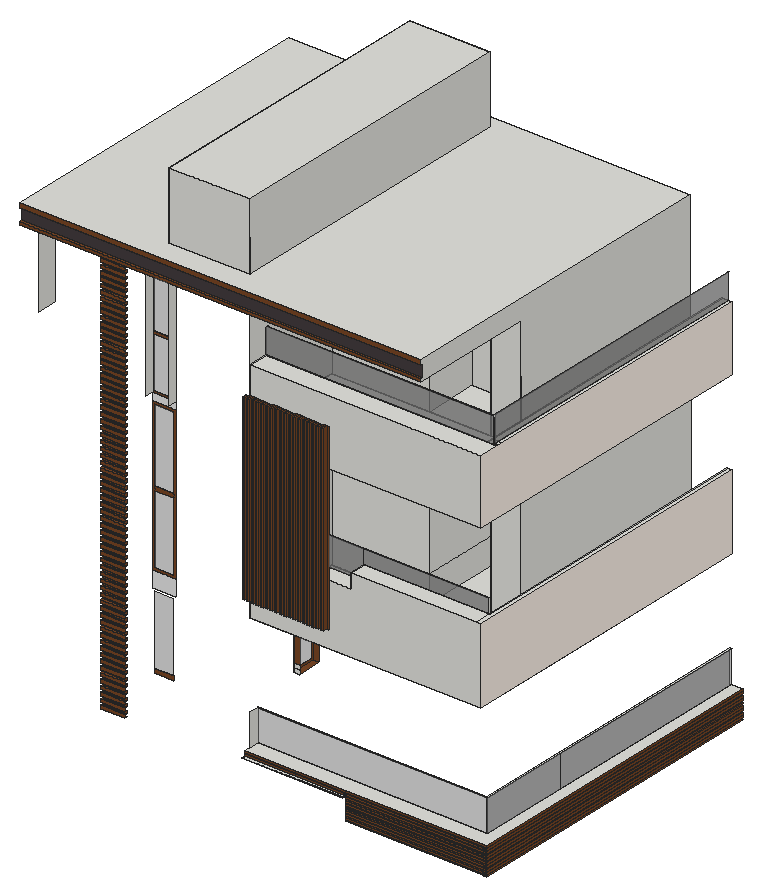
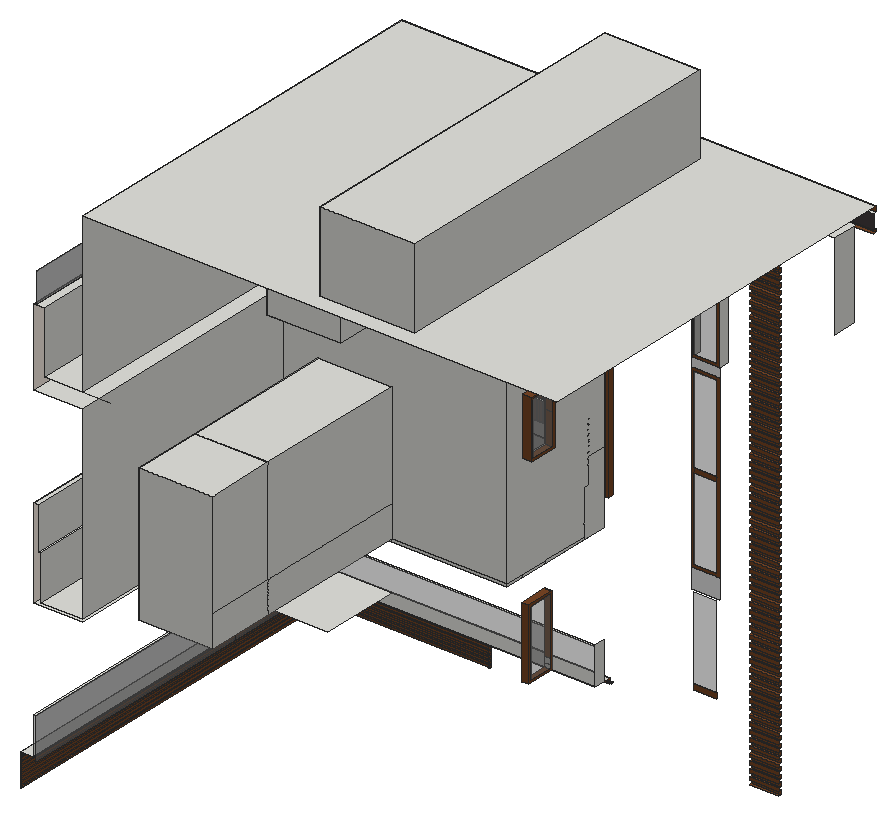
# SketchUp Ruby script. Lengths in inches.
U = 1.inch
M = Sketchup.active_model
def pt(a) = Geom::Point3d.new(a.map { |v| v * U })
def face(e, loops, mat)
  f = e.add_face(loops[0].map { |a| pt(a) })
  loops[1..].each { |l| e.add_face(l.map { |a| pt(a) }).erase! }
  f.material = f.back_material = mat if mat
  f
end
# faces: each face lists its corners as indices into pts; further lists are holes
def faces(e, pts, list, mat = nil) = list.each { |f| face(e, (f[0].is_a?(Array) ? f : [f]).map { |l| l.map { |i| pts[i] } }, mat) }
# xy, xz, yz: faces in a plane at the given z, y or x. An outline is a flat list of corners, or four numbers for a rectangle; further outlines are holes
def ring(l) = l.size == 4 ? [[l[0], l[1]], [l[2], l[1]], [l[2], l[3]], [l[0], l[3]]] : l.each_slice(2).to_a
def flat(e, list, mat, &to3) = list.each { |f| face(e, (f[0].is_a?(Array) ? f : [f]).map { |l| ring(l).map { |u, v| to3.(u, v) } }, mat) }
def xy(e, z, list, mat = nil) = flat(e, list, mat) { |x, y| [x, y, z] }
def xz(e, y, list, mat = nil) = flat(e, list, mat) { |x, z| [x, y, z] }
def yz(e, x, list, mat = nil) = flat(e, list, mat) { |y, z| [x, y, z] }
def lines(e, pts, list) = list.each { |a, b| e.add_line(pt(pts[a]), pt(pts[b])) }
# prism: a flat outline (further loops are holes) pulled along v
def prism(e, loops, v, mat = nil)
  f = face(e, loops, mat); d = Geom::Vector3d.new(v.map { |x| x * U })
  f.pushpull(f.normal.samedirection?(d) ? d.length : -d.length)
end
def box(e, o, s, mat = nil) = prism(e, [[o, [o[0] + s[0], o[1], o[2]], [o[0] + s[0], o[1] + s[1], o[2]], [o[0], o[1] + s[1], o[2]]]], [0, 0, s[2]], mat)
def at(x, y, z, deg = 0) = Geom::Transformation.translation(pt([x, y, z])) * Geom::Transformation.rotation(ORIGIN, Z_AXIS, deg.degrees)
def axes(o, x, y, z) = Geom::Transformation.new([*x, 0, *y, 0, *z, 0, *pt(o).to_a, 1])
def part(name) = M.definitions.add(name)
# library, detail: a bought-in or finely detailed component or shape, given as its bounding box
def library(name, o, s) = part(name).tap { |d| box(d.entities, o, s) }
def detail(e, o, s) = box(e.add_group.entities, o, s)
def put(e, d, t, mat = nil) = e.add_instance(d, t).tap { |i| i.material = mat if mat }
def group(e, t, mat = nil) = e.add_group.tap { |g| g.transformation = t; g.material = mat if mat }.entities
root = M.entities
M.materials.add("[0009_Linen]").color = [250, 240, 230]
M.materials.add("[Asphalt New]").color = [67, 60, 62]
M.materials.add("[Polished Concrete Old]").color = [229, 229, 229]
M.materials.add("[Translucent Glass Gray]").color = [128, 128, 128]
M.materials["[Translucent Glass Gray]"].alpha = 0.5
M.materials.add("[Wood Veneer 01]").color = [120, 70, 37]
xy(root,339.5,[[701.8,342.29,960.69,342.73],[960.69,342.73,962.51,934.03]],"[Wood Veneer 01]")
xy(root,342.02,[[701.8,342.29,960.69,342.73],[960.69,342.73,962.51,934.03]],"[Wood Veneer 01]")
xy(root,343.69,[[224.18,374.04,268.36,378.04]],"[Wood Veneer 01]")
xy(root,345.19,[[701.8,342.29,960.69,342.73],[960.69,342.73,962.51,934.03]],"[Wood Veneer 01]")
xy(root,347.71,[[701.8,342.29,960.69,342.73],[960.69,342.73,962.51,934.03]],"[Wood Veneer 01]")
xy(root,349.71,[[224.18,374.04,268.36,378.04]],"[Wood Veneer 01]")
xy(root,350.88,[[701.8,342.29,960.69,342.73],[960.69,342.73,962.51,934.03]],"[Wood Veneer 01]")
xy(root,353.39,[[701.8,342.29,960.69,342.73],[960.69,342.73,962.51,934.03]],"[Wood Veneer 01]")
xy(root,354.57,[[224.18,374.04,268.36,378.04]],"[Wood Veneer 01]")
xy(root,356.57,[[701.8,342.29,960.69,342.73],[960.69,342.73,962.51,934.03]],"[Wood Veneer 01]")
xy(root,359.08,[[701.8,342.29,960.69,342.73],[960.69,342.73,962.51,934.03]],"[Wood Veneer 01]")
xy(root,360.59,[[224.18,374.04,268.36,378.04]],"[Wood Veneer 01]")
xy(root,362.25,[[701.8,342.29,960.69,342.73],[960.69,342.73,962.51,934.03]],"[Wood Veneer 01]")
xy(root,364.77,[[701.8,342.29,960.69,342.73],[960.69,342.73,962.51,934.03]],"[Wood Veneer 01]")
xy(root,365.44,[[224.18,374.04,268.36,378.04]],"[Wood Veneer 01]")
xy(root,367.94,[[701.8,342.29,960.69,342.73],[960.69,342.73,962.51,934.03]],"[Wood Veneer 01]")
xy(root,370.46,[[701.8,342.29,960.69,342.73],[960.69,342.73,962.51,934.03]],"[Wood Veneer 01]")
xy(root,371.46,[[224.18,374.04,268.36,378.04]],"[Wood Veneer 01]")
xy(root,373.63,[[701.8,342.29,960.69,342.73],[960.69,342.73,962.51,934.03]],"[Wood Veneer 01]")
xy(root,376.14,[[701.8,342.29,960.69,342.73],[960.69,342.73,962.51,934.03]],"[Wood Veneer 01]")
xy(root,376.32,[[224.18,374.04,268.36,378.04]],"[Wood Veneer 01]")
xy(root,379.32,[[701.8,342.29,960.69,342.73],[960.69,342.73,962.51,934.03]],"[Wood Veneer 01]")
xy(root,380.42,[[515.24,336.73,701.8,339.61]])
xy(root,381.83,[[515.24,336.73,701.8,342.29]])
xy(root,381.83,[[701.8,342.29,960.69,342.73],[960.69,342.73,962.51,934.03]],"[Wood Veneer 01]")
xy(root,382.34,[[224.18,374.04,268.36,378.04]],"[Wood Veneer 01]")
xy(root,385,[[515.24,342.29,701.8,342.73],[701.8,342.29,960.69,342.73],[960.69,342.73,962.51,934.03]],"[Wood Veneer 01]")
xy(root,386.71,[[515.24,342.29,701.8,342.73],[701.8,342.29,962.51,342.73],[960.69,342.73,962.51,934.03]],"[Wood Veneer 01]")
xy(root,387.19,[[224.18,374.04,268.36,378.04]],"[Wood Veneer 01]")
xy(root,390.25,[[515.24,342.29,962.51,342.29,962.51,934.03,941.71,934.03,941.71,371.82,515.24,371.82]])
xy(root,393.21,[[224.18,374.04,268.36,378.04]],"[Wood Veneer 01]")
xy(root,398.07,[[224.18,374.04,268.36,378.04]],"[Wood Veneer 01]")
xy(root,404.09,[[224.18,374.04,268.36,378.04]],"[Wood Veneer 01]")
xy(root,408.94,[[224.18,374.04,268.36,378.04]],"[Wood Veneer 01]")
xy(root,414.96,[[224.18,374.04,268.36,378.04]],"[Wood Veneer 01]")
xy(root,419.82,[[224.18,374.04,268.36,378.04]],"[Wood Veneer 01]")
xy(root,425.84,[[224.18,374.04,268.36,378.04]],"[Wood Veneer 01]")
xy(root,430.69,[[224.18,374.04,268.36,378.04]],"[Wood Veneer 01]")
xy(root,436.71,[[224.18,374.04,268.36,378.04]],"[Wood Veneer 01]")
xy(root,441.57,[[224.18,374.04,268.36,378.04]],"[Wood Veneer 01]")
xy(root,447.59,[[224.18,374.04,268.36,378.04]],"[Wood Veneer 01]")
xy(root,449.0625,[[515.24,371.82,941.71,371.82,941.71,934.03,937.99,934.03,937.99,373.53,515.24,373.53]])
xy(root,452.44,[[224.18,374.04,268.36,378.04]],"[Wood Veneer 01]")
xy(root,458.46,[[224.18,374.04,268.36,378.04]],"[Wood Veneer 01]")
xy(root,461.11,[[504.05,469.55,515.24,514.92]],"[Wood Veneer 01]")
xy(root,463.32,[[224.18,374.04,268.36,378.04]],"[Wood Veneer 01]")
xy(root,469.34,[[224.18,374.04,268.36,378.04]],"[Wood Veneer 01]")
xy(root,474.19,[[224.18,374.04,268.36,378.04]],"[Wood Veneer 01]")
xy(root,480.21,[[224.18,374.04,268.36,378.04]],"[Wood Veneer 01]")
xy(root,485.07,[[224.18,374.04,268.36,378.04]],"[Wood Veneer 01]")
xy(root,491.09,[[224.18,374.04,268.36,378.04]],"[Wood Veneer 01]")
xy(root,495.94,[[224.18,374.04,268.36,378.04]],"[Wood Veneer 01]")
xy(root,501.96,[[224.18,374.04,268.36,378.04]],"[Wood Veneer 01]")
xy(root,507.44,[[224.18,374.04,268.36,378.04]],"[Wood Veneer 01]")
xy(root,513.46,[[224.18,374.04,268.36,378.04]],"[Wood Veneer 01]")
xy(root,518.94,[[224.18,374.04,268.36,378.04]],"[Wood Veneer 01]")
xy(root,524.96,[[224.18,374.04,268.36,378.04]],"[Wood Veneer 01]")
xy(root,530.44,[[224.18,374.04,268.36,378.04]],"[Wood Veneer 01]")
xy(root,534.49,[[695.625,543.54,810.09,667.11]])
xy(root,536.46,[[224.18,374.04,268.36,378.04]],"[Wood Veneer 01]")
xy(root,541.94,[[224.18,374.04,268.36,378.04]],"[Wood Veneer 01]")
xy(root,547.96,[[224.18,374.04,268.36,378.04]],"[Wood Veneer 01]")
xy(root,553.44,[[224.18,374.04,268.36,378.04]],"[Wood Veneer 01]")
xy(root,559.46,[[224.18,374.04,268.36,378.04]],"[Wood Veneer 01]")
xy(root,564.94,[[224.18,374.04,268.36,378.04]],"[Wood Veneer 01]")
xy(root,570.96,[[224.18,374.04,268.36,378.04]],"[Wood Veneer 01]")
xy(root,571.62,[[504.05,469.55,515.24,514.92]],"[Wood Veneer 01]")
xy(root,576.44,[[224.18,374.04,268.36,378.04]],"[Wood Veneer 01]")
xy(root,582.46,[[224.18,374.04,268.36,378.04]],"[Wood Veneer 01]")
xy(root,587.94,[[224.18,374.04,268.36,378.04]],"[Wood Veneer 01]")
xy(root,593.96,[[224.18,374.04,268.36,378.04]],"[Wood Veneer 01]")
xy(root,599.44,[[224.18,374.04,268.36,378.04]],"[Wood Veneer 01]")
xy(root,605.46,[[224.18,374.04,268.36,378.04]],"[Wood Veneer 01]")
xy(root,605.77,[[865.61,543.54,941.71,934.03]])
xy(root,605.77,[[515.24,354.61,941.71,543.54]],"[Wood Veneer 01]")
xy(root,609.59,[[515.24,394.39,930.23,394.39,930.23,934.03,865.61,934.03,865.61,543.54,515.24,543.54],[695.625,543.54,810.09,783.98],[695.625,783.98,810.09,892.86]])
xy(root,610.94,[[224.18,374.04,268.36,378.04]],"[Wood Veneer 01]")
xy(root,616.96,[[224.18,374.04,268.36,378.04]],"[Wood Veneer 01]")
xy(root,622.44,[[224.18,374.04,268.36,378.04]],"[Wood Veneer 01]")
xy(root,628.46,[[224.18,374.04,268.36,378.04]],"[Wood Veneer 01]")
xy(root,633.94,[[224.18,374.04,268.36,378.04]],"[Wood Veneer 01]")
xy(root,639.96,[[224.18,374.04,268.36,378.04]],"[Wood Veneer 01]")
xy(root,645.44,[[224.18,374.04,268.36,378.04]],"[Wood Veneer 01]")
xy(root,651.46,[[224.18,374.04,268.36,378.04]],"[Wood Veneer 01]")
xy(root,656.94,[[224.18,374.04,268.36,378.04]],"[Wood Veneer 01]")
xy(root,662.96,[[224.18,374.04,268.36,378.04]],"[Wood Veneer 01]")
xy(root,668.44,[[224.18,374.04,268.36,378.04]],"[Wood Veneer 01]")
xy(root,674.46,[[224.18,374.04,268.36,378.04]],"[Wood Veneer 01]")
xy(root,679.4,[[515.24,385.86,933.62,385.86,933.62,934.03,930.23,934.03,930.23,394.39,515.24,394.39]])
xy(root,679.94,[[224.18,374.04,268.36,378.04]],"[Wood Veneer 01]")
xy(root,685.96,[[224.18,374.04,268.36,378.04]],"[Wood Veneer 01]")
xy(root,691.44,[[224.18,374.04,268.36,378.04]],"[Wood Veneer 01]")
xy(root,697.46,[[224.18,374.04,268.36,378.04]],"[Wood Veneer 01]")
xy(root,702.94,[[224.18,374.04,268.36,378.04]],"[Wood Veneer 01]")
xy(root,708.96,[[224.18,374.04,268.36,378.04]],"[Wood Veneer 01]")
xy(root,714.44,[[224.18,374.04,268.36,378.04]],"[Wood Veneer 01]")
xy(root,718.96,[[515.24,354.61,701.8,383.52]])
xy(root,720.46,[[224.18,374.04,268.36,378.04]],"[Wood Veneer 01]")
xy(root,725.94,[[224.18,374.04,268.36,378.04]],"[Wood Veneer 01]")
xy(root,731.96,[[224.18,374.04,268.36,378.04]],"[Wood Veneer 01]")
xy(root,737.44,[[224.18,374.04,268.36,378.04]],"[Wood Veneer 01]")
xy(root,743.46,[[224.18,374.04,268.36,378.04]],"[Wood Veneer 01]")
xy(root,745.21,[[701.8,354.61,933.62,383.52],[933.62,354.61,941.71,934.03]])
xy(root,748.94,[[224.18,374.04,268.36,378.04]],"[Wood Veneer 01]")
xy(root,754.96,[[224.18,374.04,268.36,378.04]],"[Wood Veneer 01]")
xy(root,760.44,[[224.18,374.04,268.36,378.04]],"[Wood Veneer 01]")
xy(root,766.46,[[224.18,374.04,268.36,378.04]],"[Wood Veneer 01]")
xy(root,771.94,[[224.18,374.04,268.36,378.04]],"[Wood Veneer 01]")
xy(root,772.09,[[515.24,383.52,933.62,385.86]])
xy(root,773.36,[[500.24,469.55,515.24,514.92]],"[Wood Veneer 01]")
xy(root,777.96,[[224.18,374.04,268.36,378.04]],"[Wood Veneer 01]")
xy(root,783.44,[[224.18,374.04,268.36,378.04]],"[Wood Veneer 01]")
xy(root,789.46,[[224.18,374.04,268.36,378.04]],"[Wood Veneer 01]")
xy(root,794.94,[[224.18,374.04,268.36,378.04]],"[Wood Veneer 01]")
xy(root,800.96,[[224.18,374.04,268.36,378.04]],"[Wood Veneer 01]")
xy(root,806.44,[[224.18,374.04,268.36,378.04]],"[Wood Veneer 01]")
xy(root,812.46,[[224.18,374.04,268.36,378.04]],"[Wood Veneer 01]")
xy(root,817.94,[[224.18,374.04,268.36,378.04]],"[Wood Veneer 01]")
xy(root,822.42,[[695.625,543.54,810.09,783.98],[695.625,783.98,810.09,892.86]])
xy(root,823.96,[[224.18,374.04,268.36,378.04]],"[Wood Veneer 01]")
xy(root,829.44,[[224.18,374.04,268.36,378.04]],"[Wood Veneer 01]")
xy(root,835.46,[[224.18,374.04,268.36,378.04]],"[Wood Veneer 01]")
xy(root,840.94,[[224.18,374.04,268.36,378.04]],"[Wood Veneer 01]")
xy(root,846.96,[[224.18,374.04,268.36,378.04]],"[Wood Veneer 01]")
xy(root,851.5,[[224.18,374.04,268.36,378.04]],"[Wood Veneer 01]")
xy(root,857.52,[[224.18,374.04,268.36,378.04]],"[Wood Veneer 01]")
xy(root,862.07,[[224.18,374.04,268.36,378.04]],"[Wood Veneer 01]")
xy(root,862.63,[[500.24,469.55,515.24,514.92]],"[Wood Veneer 01]")
xy(root,868.09,[[224.18,374.04,268.36,378.04]],"[Wood Veneer 01]")
xy(root,872.63,[[224.18,374.04,268.36,378.04]],"[Wood Veneer 01]")
xy(root,878.65,[[224.18,374.04,268.36,378.04]],"[Wood Veneer 01]")
xy(root,883.19,[[224.18,374.04,268.36,378.04]],"[Wood Veneer 01]")
xy(root,889.21,[[224.18,374.04,268.36,378.04]],"[Wood Veneer 01]")
xy(root,893.75,[[224.18,374.04,268.36,378.04]],"[Wood Veneer 01]")
xy(root,899.77,[[224.18,374.04,268.36,378.04]],"[Wood Veneer 01]")
xy(root,903.4375,[[865.61,543.54,941.71,934.03]])
xy(root,903.4375,[[515.24,354.61,941.71,543.54]],"[Wood Veneer 01]")
xy(root,904.32,[[224.18,374.04,268.36,378.04]],"[Wood Veneer 01]")
xy(root,910.34,[[224.18,374.04,268.36,378.04]],"[Wood Veneer 01]")
xy(root,914.88,[[224.18,374.04,268.36,378.04]],"[Wood Veneer 01]")
xy(root,920.9,[[224.18,374.04,268.36,378.04]],"[Wood Veneer 01]")
xy(root,925.44,[[224.18,374.04,268.36,378.04]],"[Wood Veneer 01]")
xy(root,926.8125,[[515.24,392.01,924.26,392.01,924.26,934.03,865.53,934.03,865.53,543.54,515.24,543.54],[695.625,543.54,810.09,642.86]])
xy(root,931.46,[[224.18,374.04,268.36,378.04]],"[Wood Veneer 01]")
xy(root,936,[[224.18,374.04,268.36,378.04]],"[Wood Veneer 01]")
xy(root,942.02,[[224.18,374.04,268.36,378.04]],"[Wood Veneer 01]")
xy(root,946.57,[[224.18,374.04,268.36,378.04]],"[Wood Veneer 01]")
xy(root,952.59,[[224.18,374.04,268.36,378.04]],"[Wood Veneer 01]")
xy(root,957.13,[[224.18,374.04,268.36,378.04]],"[Wood Veneer 01]")
xy(root,963.15,[[224.18,374.04,268.36,378.04]],"[Wood Veneer 01]")
xy(root,967.69,[[224.18,374.04,268.36,378.04]],"[Wood Veneer 01]")
xy(root,973.71,[[224.18,374.04,268.36,378.04]],"[Wood Veneer 01]")
xy(root,978.25,[[224.18,374.04,268.36,378.04]],"[Wood Veneer 01]")
xy(root,984.27,[[224.18,374.04,268.36,378.04]],"[Wood Veneer 01]")
xy(root,988.82,[[224.18,374.04,268.36,378.04]],"[Wood Veneer 01]")
xy(root,994.84,[[224.18,374.04,268.36,378.04]],"[Wood Veneer 01]")
xy(root,999.38,[[224.18,374.04,268.36,378.04]],"[Wood Veneer 01]")
xy(root,1005.4,[[224.18,374.04,268.36,378.04]],"[Wood Veneer 01]")
xy(root,1009.94,[[224.18,374.04,268.36,378.04]],"[Wood Veneer 01]")
xy(root,1015.96,[[224.18,374.04,268.36,378.04]],"[Wood Veneer 01]")
xy(root,1020.5,[[224.18,374.04,268.36,378.04]],"[Wood Veneer 01]")
xy(root,1023.625,[[515.24,354.61,941.71,391.73],[936.87,391.73,941.71,393.38],[924.26,392.01,936.15,402.93],[936.87,393.38,941.71,402.93],[924.26,402.93,936.15,934.03],
  [936.87,402.93,941.71,934.03]])
xy(root,1026.52,[[224.18,374.04,268.36,378.04]],"[Wood Veneer 01]")
xy(root,1031.07,[[224.18,374.04,268.36,378.04]],"[Wood Veneer 01]")
xy(root,1031.82,[[501.05,469.55,515.24,514.92]],"[Wood Veneer 01]")
xy(root,1037.09,[[224.18,374.04,268.36,378.04]],"[Wood Veneer 01]")
xy(root,1041.63,[[224.18,374.04,268.36,378.04]],"[Wood Veneer 01]")
xy(root,1047.65,[[224.18,374.04,268.36,378.04]],"[Wood Veneer 01]")
xy(root,1052.19,[[224.18,374.04,268.36,378.04]],"[Wood Veneer 01]")
xy(root,1058.21,[[224.18,374.04,268.36,378.04]],"[Wood Veneer 01]")
xy(root,1062.75,[[224.18,374.04,268.36,378.04]],"[Wood Veneer 01]")
xy(root,1068.77,[[224.18,374.04,268.36,378.04]],"[Wood Veneer 01]")
xy(root,1071.875,[[515.24,391.73,936.87,391.73,936.87,393.38,936.15,393.38,936.15,392.01,515.24,392.01],[936.15,393.38,936.87,934.03]])
xy(root,1073.32,[[224.18,374.04,268.36,378.04]],"[Wood Veneer 01]")
xy(root,1079.34,[[224.18,374.04,268.36,378.04]],"[Wood Veneer 01]")
xy(root,1083.88,[[224.18,374.04,268.36,378.04]],"[Wood Veneer 01]")
xy(root,1089.9,[[224.18,374.04,268.36,378.04]],"[Wood Veneer 01]")
xy(root,1094.44,[[224.18,374.04,268.36,378.04]],"[Wood Veneer 01]")
xy(root,1100.46,[[224.18,374.04,268.36,378.04]],"[Wood Veneer 01]")
xy(root,1105,[[224.18,374.04,268.36,378.04]],"[Wood Veneer 01]")
xy(root,1111.02,[[224.18,374.04,268.36,378.04]],"[Wood Veneer 01]")
xy(root,1115.76,[[224.18,374.04,268.36,378.04]],"[Wood Veneer 01]")
xy(root,1120.01,[[501.05,469.55,515.24,514.92]],"[Wood Veneer 01]")
xy(root,1120.3,[[224.18,374.04,268.36,378.04]],"[Wood Veneer 01]")
xy(root,1124.95,[[224.18,374.04,268.36,378.04]],"[Wood Veneer 01]")
xy(root,1129.68,[[224.18,374.04,268.36,378.04]],"[Wood Veneer 01]")
xy(root,1137.19,[[154.8,311.67,154.8,354.61,224.18,354.61,224.18,378.04,268.36,378.04,268.36,354.61,322.47,354.61,322.47,370.17,366.22,370.17,366.22,354.61,515.24,354.61,515.24,311.67]])
xy(root,1137.19,[[124.44,311.67,154.8,316.98],[515.24,311.67,865.53,543.54]],"[Wood Veneer 01]")
xy(root,1142.63,[[124.44,311.67,865.53,316.98]],"[Wood Veneer 01]")
xy(root,1165.85,[[124.44,311.67,865.53,316.98]])
xy(root,1173.6875,[[[124.44,311.67,865.53,934.03],[366.22,354.61,514.47,909.23]]])
xy(root,1298.375,[[366.22,354.61,514.47,909.23]])
xz(root,311.67,[[124.44,1137.19,865.53,1142.63],[124.44,1165.85,865.53,1173.6875]],"[Wood Veneer 01]")
xz(root,316.98,[[124.44,1142.63,865.53,1165.85]],"[Asphalt New]")
xz(root,336.73,[[515.24,380.42,701.8,381.83]],"[Polished Concrete Old]")
xz(root,342.29,[[701.8,342.02,960.69,345.19],[701.8,347.71,960.69,350.88],[701.8,353.39,960.69,356.57],[701.8,359.08,960.69,362.25],[701.8,364.77,960.69,367.94],
  [701.8,370.46,960.69,373.63],[701.8,376.14,960.69,379.32],[515.24,381.83,701.8,385],[701.8,381.83,960.69,385],[515.24,386.71,701.8,390.25],
  [701.8,386.71,962.51,390.25]],"[Wood Veneer 01]")
xz(root,342.73,[[701.8,381.83,960.69,385]])
xz(root,342.73,[[701.8,339.5,960.69,342.02],[960.69,342.02,962.51,345.19],[701.8,345.19,960.69,347.71],[960.69,347.71,962.51,350.88],[701.8,350.88,960.69,353.39],
  [960.69,353.39,962.51,356.57],[701.8,356.57,960.69,359.08],[960.69,359.08,962.51,362.25],[701.8,362.25,960.69,364.77],[960.69,364.77,962.51,367.94],
  [701.8,367.94,960.69,370.46],[960.69,370.46,962.51,373.63],[701.8,373.63,960.69,376.14],[960.69,376.14,962.51,379.32],[701.8,379.32,960.69,381.83],
  [960.69,381.83,962.51,385],[515.24,385,701.8,386.71],[701.8,385,960.69,386.71]],"[Wood Veneer 01]")
xz(root,354.61,[[515.24,605.77,941.71,605.77,941.71,745.21,701.8,745.21,701.8,718.96,515.24,718.96],[515.24,903.4375,941.71,1023.625],[366.22,1173.6875,514.47,1298.375]])
xz(root,370.17,[[322.47,579.93,366.22,610.32],[322.47,889.77,366.22,904.26]],"[Polished Concrete Old]")
xz(root,370.17,[[326.19,448.15,362.49,576.21],[326.54,614.39,362.14,742.65],[326.54,750.04,362.14,885.69],[325.93,907.72,362.75,1002.17],[325.93,1007.32,362.75,1106.93]],"[Translucent Glass Gray]")
xz(root,370.17,[[326.19,440.01,362.49,448.15],[[322.47,610.32,366.22,889.77],[326.54,614.39,362.14,885.69]],[326.54,742.65,362.14,750.04],[[322.47,904.26,366.22,1111.14],[325.93,907.72,362.75,1106.93]],[325.93,1002.17,362.75,1007.32],
  [322.47,1111.14,366.22,1133.73],[322.47,1133.73,366.22,1137.19]],"[Wood Veneer 01]")
xz(root,371.82,[[515.24,390.25,941.71,449.0625]],"[Translucent Glass Gray]")
xz(root,374.04,[[224.18,343.69,268.36,349.71],[224.18,354.57,268.36,360.59],[224.18,365.44,268.36,371.46],[224.18,376.32,268.36,382.34],[224.18,387.19,268.36,393.21],
  [224.18,398.07,268.36,404.09],[224.18,408.94,268.36,414.96],[224.18,419.82,268.36,425.84],[224.18,430.69,268.36,436.71],[224.18,441.57,268.36,447.59],
  [224.18,452.44,268.36,458.46],[224.18,463.32,268.36,469.34],[224.18,474.19,268.36,480.21],[224.18,485.07,268.36,491.09],[224.18,495.94,268.36,501.96],
  [224.18,507.44,268.36,513.46],[224.18,518.94,268.36,524.96],[224.18,530.44,268.36,536.46],[224.18,541.94,268.36,547.96],[224.18,553.44,268.36,559.46],
  [224.18,564.94,268.36,570.96],[224.18,576.44,268.36,582.46],[224.18,587.94,268.36,593.96],[224.18,599.44,268.36,605.46],[224.18,610.94,268.36,616.96],
  [224.18,622.44,268.36,628.46],[224.18,633.94,268.36,639.96],[224.18,645.44,268.36,651.46],[224.18,656.94,268.36,662.96],[224.18,668.44,268.36,674.46],
  [224.18,679.94,268.36,685.96],[224.18,691.44,268.36,697.46],[224.18,702.94,268.36,708.96],[224.18,714.44,268.36,720.46],[224.18,725.94,268.36,731.96],
  [224.18,737.44,268.36,743.46],[224.18,748.94,268.36,754.96],[224.18,760.44,268.36,766.46],[224.18,771.94,268.36,777.96],[224.18,783.44,268.36,789.46],
  [224.18,794.94,268.36,800.96],[224.18,806.44,268.36,812.46],[224.18,817.94,268.36,823.96],[224.18,829.44,268.36,835.46],[224.18,840.94,268.36,846.96],
  [224.18,851.5,268.36,857.52],[224.18,862.07,268.36,868.09],[224.18,872.63,268.36,878.65],[224.18,883.19,268.36,889.21],[224.18,893.75,268.36,899.77],
  [224.18,904.32,268.36,910.34],[224.18,914.88,268.36,920.9],[224.18,925.44,268.36,931.46],[224.18,936,268.36,942.02],[224.18,946.57,268.36,952.59],
  [224.18,957.13,268.36,963.15],[224.18,967.69,268.36,973.71],[224.18,978.25,268.36,984.27],[224.18,988.82,268.36,994.84],[224.18,999.38,268.36,1005.4],
  [224.18,1009.94,268.36,1015.96],[224.18,1020.5,268.36,1026.52],[224.18,1031.07,268.36,1037.09],[224.18,1041.63,268.36,1047.65],[224.18,1052.19,268.36,1058.21],
  [224.18,1062.75,268.36,1068.77],[224.18,1073.32,268.36,1079.34],[224.18,1083.88,268.36,1089.9],[224.18,1094.44,268.36,1100.46],[224.18,1105,268.36,1111.02],
  [224.18,1115.76,268.36,1120.3],[224.18,1124.95,268.36,1129.68]],"[Wood Veneer 01]")
xz(root,378.04,[[224.18,349.71,268.36,354.57],[224.18,360.59,268.36,365.44],[224.18,371.46,268.36,376.32],[224.18,382.34,268.36,387.19],[224.18,393.21,268.36,398.07],
  [224.18,404.09,268.36,408.94],[224.18,414.96,268.36,419.82],[224.18,425.84,268.36,430.69],[224.18,436.71,268.36,441.57],[224.18,447.59,268.36,452.44],
  [224.18,458.46,268.36,463.32],[224.18,469.34,268.36,474.19],[224.18,480.21,268.36,485.07],[224.18,491.09,268.36,495.94],[224.18,501.96,268.36,507.44],
  [224.18,513.46,268.36,518.94],[224.18,524.96,268.36,530.44],[224.18,536.46,268.36,541.94],[224.18,547.96,268.36,553.44],[224.18,559.46,268.36,564.94],
  [224.18,570.96,268.36,576.44],[224.18,582.46,268.36,587.94],[224.18,593.96,268.36,599.44],[224.18,605.46,268.36,610.94],[224.18,616.96,268.36,622.44],
  [224.18,628.46,268.36,633.94],[224.18,639.96,268.36,645.44],[224.18,651.46,268.36,656.94],[224.18,662.96,268.36,668.44],[224.18,674.46,268.36,679.94],
  [224.18,685.96,268.36,691.44],[224.18,697.46,268.36,702.94],[224.18,708.96,268.36,714.44],[224.18,720.46,268.36,725.94],[224.18,731.96,268.36,737.44],
  [224.18,743.46,268.36,748.94],[224.18,754.96,268.36,760.44],[224.18,766.46,268.36,771.94],[224.18,777.96,268.36,783.44],[224.18,789.46,268.36,794.94],
  [224.18,800.96,268.36,806.44],[224.18,812.46,268.36,817.94],[224.18,823.96,268.36,829.44],[224.18,835.46,268.36,840.94],[224.18,846.96,268.36,851.5],
  [224.18,857.52,268.36,862.07],[224.18,868.09,268.36,872.63],[224.18,878.65,268.36,883.19],[224.18,889.21,268.36,893.75],[224.18,899.77,268.36,904.32],
  [224.18,910.34,268.36,914.88],[224.18,920.9,268.36,925.44],[224.18,931.46,268.36,936],[224.18,942.02,268.36,946.57],[224.18,952.59,268.36,957.13],
  [224.18,963.15,268.36,967.69],[224.18,973.71,268.36,978.25],[224.18,984.27,268.36,988.82],[224.18,994.84,268.36,999.38],[224.18,1005.4,268.36,1009.94],
  [224.18,1015.96,268.36,1020.5],[224.18,1026.52,268.36,1031.07],[224.18,1037.09,268.36,1041.63],[224.18,1047.65,268.36,1052.19],[224.18,1058.21,268.36,1062.75],
  [224.18,1068.77,268.36,1073.32],[224.18,1079.34,268.36,1083.88],[224.18,1089.9,268.36,1094.44],[224.18,1100.46,268.36,1105],[224.18,1111.02,268.36,1115.76],
  [224.18,1120.3,268.36,1124.95],[224.18,1129.68,268.36,1137.19]],"[Wood Veneer 01]")
xz(root,383.52,[[515.24,718.96,701.8,772.09],[701.8,745.21,933.62,772.09]],"[Translucent Glass Gray]")
xz(root,385.86,[[515.24,679.4,933.62,772.09]],"[Translucent Glass Gray]")
xz(root,391.73,[[515.24,1023.625,936.87,1071.875]],"[Translucent Glass Gray]")
xz(root,392.01,[[515.24,926.8125,924.26,1023.625]])
xz(root,392.01,[[515.24,1023.625,936.15,1071.875]],"[Translucent Glass Gray]")
xz(root,394.39,[[515.24,609.59,930.23,679.4]])
xz(root,469.55,[[504.05,461.11,515.24,467.98],[504.05,467.98,515.24,476.73]])
xz(root,469.55,[[504.05,476.73,515.24,571.62],[500.24,773.36,515.24,821.82],[500.24,821.82,515.24,862.63],[501.05,1031.82,515.24,1120.01]],"[Wood Veneer 01]")
xz(root,514.92,[[504.05,461.11,515.24,571.62],[500.24,773.36,515.24,862.63],[501.05,1031.82,515.24,1120.01]],"[Wood Veneer 01]")
xz(root,543.54,[[515.24,605.77,695.625,609.59],[695.625,605.77,810.09,609.59],[810.09,605.77,865.61,609.59],[515.24,609.59,695.625,609.59,695.625,822.42,810.09,822.42,810.09,609.59,865.61,609.59,865.61,903.4375,515.24,903.4375],[515.24,903.4375,695.625,926.8125],
  [695.625,903.4375,810.09,926.8125],[515.24,926.8125,695.625,926.8125,695.625,1097.11,810.09,1096.06,810.09,926.8125,865.53,926.8125,865.53,1137.19,515.24,1137.19]])
xz(root,642.86,[[695.625,926.8125,810.09,926.8125,810.09,1096.06,695.625,1097.11]])
xz(root,783.98,[[695.625,609.59,810.09,822.42]])
xz(root,892.86,[[695.625,609.59,810.09,822.42]])
xz(root,909.23,[[366.22,1173.6875,514.47,1298.375]])
yz(root,154.8,[[316.98,1001.72,354.61,1137.19]])
yz(root,322.47,[[354.61,904.26,370.17,1137.19]])
yz(root,366.22,[[354.61,904.26,370.17,1137.19],[354.61,1173.6875,909.23,1298.375]])
yz(root,500.24,[[472.12,775.93,512.35,860.06]],"[Translucent Glass Gray]")
yz(root,500.24,[[[469.55,773.36,514.92,862.63],[472.12,775.93,512.35,860.06]]],"[Wood Veneer 01]")
yz(root,501.05,[[473.26,1035.53,511.21,1116.29]],"[Translucent Glass Gray]")
yz(root,501.05,[[[469.55,1031.82,514.92,1120.01],[473.26,1035.53,511.21,1116.29]]],"[Wood Veneer 01]")
yz(root,504.05,[[472.66,464.22,511.81,568.5]],"[Translucent Glass Gray]")
yz(root,504.05,[[[469.55,461.11,514.92,571.62],[472.66,464.22,511.81,568.5]]],"[Wood Veneer 01]")
yz(root,514.47,[[354.61,1173.6875,909.23,1298.375]])
yz(root,515.24,[[354.61,390.25,371.82,449.0625],[354.61,605.77,394.39,605.77,394.39,679.4,385.86,679.4,385.86,772.09,383.52,772.09,383.52,718.96,354.61,718.96],[394.39,605.77,469.55,609.59],[469.55,605.77,514.92,609.59],[514.92,605.77,543.54,609.59],
  [[394.39,609.59,543.54,609.59,543.54,903.4375,354.61,903.4375,354.61,718.96,383.52,718.96,383.52,772.09,385.86,772.09,385.86,679.4,394.39,679.4],[469.55,773.36,514.92,862.63]],[354.61,903.4375,354.61,1023.625,391.73,1023.625,391.73,1071.875,392.01,1071.875,392.01,926.8125,469.55,926.8125,469.55,903.4375],[469.55,903.4375,514.92,926.8125],[514.92,903.4375,543.54,926.8125],[[392.01,926.8125,543.54,926.8125,543.54,1137.19,354.61,1137.19,354.61,1023.625,391.73,1023.625,391.73,1071.875,392.01,1071.875],[469.55,1031.82,514.92,1120.01]]])
yz(root,695.625,[[543.54,609.59,783.98,658.61],[783.98,609.59,892.86,658.61],[543.54,658.61,783.98,822.42],[783.98,658.61,892.86,822.42],[543.54,926.8125,642.86,1097.11]])
yz(root,701.8,[[336.73,380.42,342.73,381.83],[354.61,718.96,383.52,745.21]])
yz(root,701.8,[[342.29,381.83,342.73,385]],"[Wood Veneer 01]")
yz(root,810.09,[[543.54,609.59,783.98,822.42],[783.98,609.59,892.86,706.18],[783.98,706.18,892.86,802.78],[783.98,802.78,892.86,822.42],[543.54,926.8125,642.86,1096.06]])
yz(root,865.53,[[543.54,926.8125,934.03,926.8125,934.03,1173.6875,311.67,1173.6875,311.67,1165.85,316.98,1165.85,316.98,1142.63,311.67,1142.63,311.67,1137.19,543.54,1137.19]])
yz(root,865.61,[[543.54,609.59,934.03,903.4375]])
yz(root,924.26,[[392.01,926.8125,934.03,1023.625]])
yz(root,930.23,[[394.39,609.59,934.03,679.4]])
yz(root,933.62,[[383.52,679.4,385.86,745.21],[385.86,679.4,934.03,745.21],[383.52,745.21,385.86,772.09]])
yz(root,936.15,[[392.01,1023.625,934.03,1071.875]],"[Translucent Glass Gray]")
yz(root,936.87,[[391.73,1023.625,393.38,1071.875]])
yz(root,936.87,[[393.38,1023.625,934.03,1071.875]],"[Translucent Glass Gray]")
yz(root,937.99,[[373.53,382.72,543.54,449.0625],[543.54,382.72,934.03,449.0625]],"[Translucent Glass Gray]")
yz(root,941.71,[[354.61,605.77,934.03,745.21],[354.61,903.4375,934.03,1023.625]],"[0009_Linen]")
yz(root,941.71,[[371.82,390.25,934.03,449.0625]],"[Translucent Glass Gray]")
yz(root,960.69,[[342.29,342.02,342.73,345.19],[342.29,347.71,342.73,350.88],[342.29,353.39,342.73,356.57],[342.29,359.08,342.73,362.25],[342.29,364.77,342.73,367.94],
  [342.29,370.46,342.73,373.63],[342.29,376.14,342.73,379.32],[342.29,381.83,342.73,385]])
yz(root,960.69,[[342.73,339.5,934.03,342.02],[342.73,345.19,934.03,347.71],[342.73,350.88,934.03,353.39],[342.73,356.57,934.03,359.08],[342.73,362.25,934.03,364.77],
  [342.73,367.94,934.03,370.46],[342.73,373.63,934.03,376.14],[342.73,379.32,934.03,381.83],[342.73,385,934.03,386.71]],"[Wood Veneer 01]")
yz(root,962.51,[[342.73,342.02,934.03,345.19],[342.73,347.71,934.03,350.88],[342.73,353.39,934.03,356.57],[342.73,359.08,934.03,362.25],[342.73,364.77,934.03,367.94],
  [342.73,370.46,934.03,373.63],[342.73,376.14,934.03,379.32],[342.73,381.83,934.03,385],[342.29,386.71,934.03,390.25]],"[Wood Veneer 01]")
p = [[810.09,543.54,1096.06],[695.625,543.54,1097.11],[695.625,642.86,1097.11],[810.09,642.86,1096.06],[701.8,383.52,718.96],[701.8,383.52,705.71],
  [821.9,934.03,926.8125],[865.53,934.03,926.8125],[865.61,543.54,903.4375],[865.61,543.54,1045.25],[515.24,354.61,1137.19],[515.24,354.61,1235.77],
  [366.22,354.61,1137.19],[366.22,354.61,1173.6875]]
faces(root,p,[[0,1,2,3]])
lines(root,p,[[4,5],[6,7],[8,9],[10,11],[12,13]])
g1 = group(root,at(515.24,345.92,643.57),"[Wood Veneer 01]")
xy(g1,0,[[0,-8.625,4.76,0],[8.53,-8.625,13.29,0],[17.0625,-8.625,21.82,0],[25.59,-8.625,30.35,0],[34.125,-8.625,38.88,0],
  [42.66,-8.625,47.41,0],[51.1875,-8.625,55.94,0],[59.72,-8.625,64.48,0],[68.25,-8.625,73.01,0],[76.78,-8.625,81.54,0],
  [85.3125,-8.625,90.07,0],[93.84,-8.625,98.6,0],[102.375,-8.625,107.13,0],[110.91,-8.625,115.66,0],[119.4375,-8.625,124.19,0],
  [127.97,-8.625,132.73,0],[136.5,-8.625,141.26,0],[145.03,-8.625,149.79,0]])
xy(g1,335.27,[[0,-8.625,4.76,0],[8.53,-8.625,13.29,0],[17.0625,-8.625,21.82,0],[25.59,-8.625,30.35,0],[34.125,-8.625,38.88,0],
  [42.66,-8.625,47.41,0],[51.1875,-8.625,55.94,0],[59.72,-8.625,64.48,0],[68.25,-8.625,73.01,0],[76.78,-8.625,81.54,0],
  [85.3125,-8.625,90.07,0],[93.84,-8.625,98.6,0],[102.375,-8.625,107.13,0],[110.91,-8.625,115.66,0],[119.4375,-8.625,124.19,0],
  [127.97,-8.625,132.73,0],[136.5,-8.625,141.26,0],[145.03,-8.625,149.79,0]])
xz(g1,-8.625,[[0,0,4.76,335.27],[8.53,0,13.29,335.27],[17.0625,0,21.82,335.27],[25.59,0,30.35,335.27],[34.125,0,38.88,335.27],
  [42.66,0,47.41,335.27],[51.1875,0,55.94,335.27],[59.72,0,64.48,335.27],[68.25,0,73.01,335.27],[76.78,0,81.54,335.27],
  [85.3125,0,90.07,335.27],[93.84,0,98.6,335.27],[102.375,0,107.13,335.27],[110.91,0,115.66,335.27],[119.4375,0,124.19,335.27],
  [127.97,0,132.73,335.27],[136.5,0,141.26,335.27],[145.03,0,149.79,335.27]])
xz(g1,0,[[0,0,4.76,335.27],[4.76,0,8.53,335.27],[13.29,0,17.0625,335.27],[21.82,0,25.59,335.27],[30.35,0,34.125,335.27],
  [38.88,0,42.66,335.27],[47.41,0,51.1875,335.27],[55.94,0,59.72,335.27],[64.48,0,68.25,335.27],[73.01,0,76.78,335.27],
  [81.54,0,85.3125,335.27],[90.07,0,93.84,335.27],[98.6,0,102.375,335.27],[107.13,0,110.91,335.27],[115.66,0,119.4375,335.27],
  [124.19,0,127.97,335.27],[132.73,0,136.5,335.27],[141.26,0,145.03,335.27],[149.79,0,153.5625,335.27]])
yz(g1,0,[[-8.625,0,0,335.27]])
yz(g1,4.76,[[-8.625,0,0,335.27]])
yz(g1,8.53,[[-8.625,0,0,335.27]])
yz(g1,13.29,[[-8.625,0,0,335.27]])
yz(g1,17.0625,[[-8.625,0,0,335.27]])
yz(g1,21.82,[[-8.625,0,0,335.27]])
yz(g1,25.59,[[-8.625,0,0,335.27]])
yz(g1,30.35,[[-8.625,0,0,335.27]])
yz(g1,34.125,[[-8.625,0,0,335.27]])
yz(g1,38.88,[[-8.625,0,0,335.27]])
yz(g1,42.66,[[-8.625,0,0,335.27]])
yz(g1,47.41,[[-8.625,0,0,335.27]])
yz(g1,51.1875,[[-8.625,0,0,335.27]])
yz(g1,55.94,[[-8.625,0,0,335.27]])
yz(g1,59.72,[[-8.625,0,0,335.27]])
yz(g1,64.48,[[-8.625,0,0,335.27]])
yz(g1,68.25,[[-8.625,0,0,335.27]])
yz(g1,73.01,[[-8.625,0,0,335.27]])
yz(g1,76.78,[[-8.625,0,0,335.27]])
yz(g1,81.54,[[-8.625,0,0,335.27]])
yz(g1,85.3125,[[-8.625,0,0,335.27]])
yz(g1,90.07,[[-8.625,0,0,335.27]])
yz(g1,93.84,[[-8.625,0,0,335.27]])
yz(g1,98.6,[[-8.625,0,0,335.27]])
yz(g1,102.375,[[-8.625,0,0,335.27]])
yz(g1,107.13,[[-8.625,0,0,335.27]])
yz(g1,110.91,[[-8.625,0,0,335.27]])
yz(g1,115.66,[[-8.625,0,0,335.27]])
yz(g1,119.4375,[[-8.625,0,0,335.27]])
yz(g1,124.19,[[-8.625,0,0,335.27]])
yz(g1,127.97,[[-8.625,0,0,335.27]])
yz(g1,132.73,[[-8.625,0,0,335.27]])
yz(g1,136.5,[[-8.625,0,0,335.27]])
yz(g1,141.26,[[-8.625,0,0,335.27]])
yz(g1,145.03,[[-8.625,0,0,335.27]])
yz(g1,149.79,[[-8.625,0,0,335.27]])
